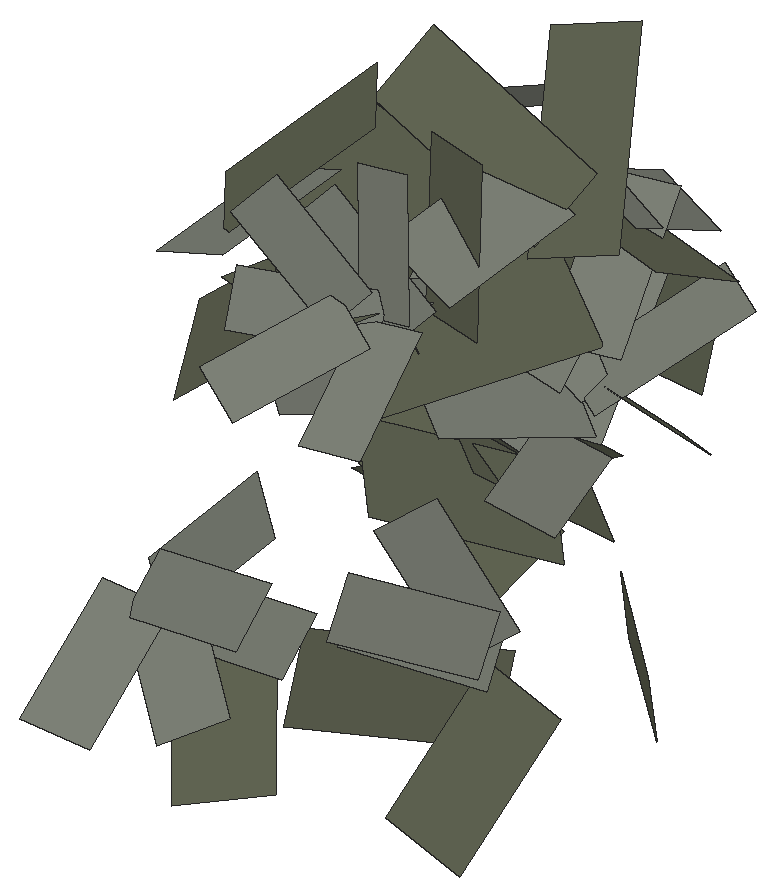
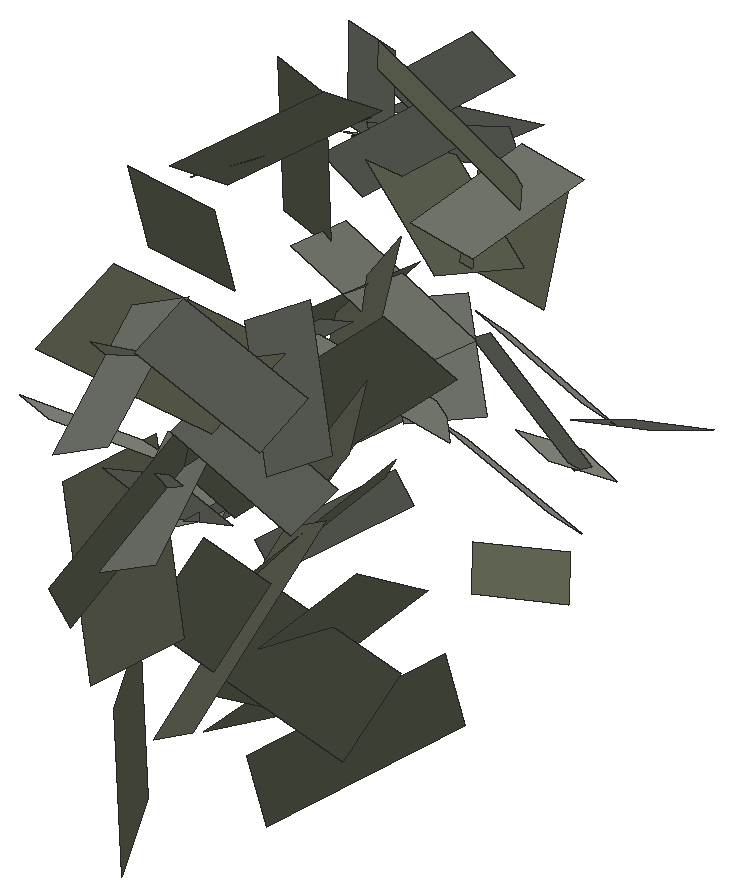
# SketchUp Ruby script. Lengths in inches.
U = 1.inch
M = Sketchup.active_model
def pt(a) = Geom::Point3d.new(a.map { |v| v * U })
def face(e, loops, mat)
  f = e.add_face(loops[0].map { |a| pt(a) })
  loops[1..].each { |l| e.add_face(l.map { |a| pt(a) }).erase! }
  f.material = f.back_material = mat if mat
  f
end
# faces: each face lists its corners as indices into pts; further lists are holes
def faces(e, pts, list, mat = nil) = list.each { |f| face(e, (f[0].is_a?(Array) ? f : [f]).map { |l| l.map { |i| pts[i] } }, mat) }
# xy, xz, yz: faces in a plane at the given z, y or x. An outline is a flat list of corners, or four numbers for a rectangle; further outlines are holes
def ring(l) = l.size == 4 ? [[l[0], l[1]], [l[2], l[1]], [l[2], l[3]], [l[0], l[3]]] : l.each_slice(2).to_a
def flat(e, list, mat, &to3) = list.each { |f| face(e, (f[0].is_a?(Array) ? f : [f]).map { |l| ring(l).map { |u, v| to3.(u, v) } }, mat) }
def xy(e, z, list, mat = nil) = flat(e, list, mat) { |x, y| [x, y, z] }
def xz(e, y, list, mat = nil) = flat(e, list, mat) { |x, z| [x, y, z] }
def yz(e, x, list, mat = nil) = flat(e, list, mat) { |y, z| [x, y, z] }
def lines(e, pts, list) = list.each { |a, b| e.add_line(pt(pts[a]), pt(pts[b])) }
# prism: a flat outline (further loops are holes) pulled along v
def prism(e, loops, v, mat = nil)
  f = face(e, loops, mat); d = Geom::Vector3d.new(v.map { |x| x * U })
  f.pushpull(f.normal.samedirection?(d) ? d.length : -d.length)
end
def box(e, o, s, mat = nil) = prism(e, [[o, [o[0] + s[0], o[1], o[2]], [o[0] + s[0], o[1] + s[1], o[2]], [o[0], o[1] + s[1], o[2]]]], [0, 0, s[2]], mat)
def at(x, y, z, deg = 0) = Geom::Transformation.translation(pt([x, y, z])) * Geom::Transformation.rotation(ORIGIN, Z_AXIS, deg.degrees)
def axes(o, x, y, z) = Geom::Transformation.new([*x, 0, *y, 0, *z, 0, *pt(o).to_a, 1])
def part(name) = M.definitions.add(name)
# library, detail: a bought-in or finely detailed component or shape, given as its bounding box
def library(name, o, s) = part(name).tap { |d| box(d.entities, o, s) }
def detail(e, o, s) = box(e.add_group.entities, o, s)
def put(e, d, t, mat = nil) = e.add_instance(d, t).tap { |i| i.material = mat if mat }
def group(e, t, mat = nil) = e.add_group.tap { |g| g.transformation = t; g.material = mat if mat }.entities
root = M.entities
M.materials.add("viburnumblaasdfas0df1w06d").color = [98, 102, 84]
M.materials.add("viburnumbladsadfasdfad0w122").color = [125, 129, 119]
c1 = part("Component\#315")
p = [[0.25,0,0],[2.05,0.01,0.35],[1.81,4.2,1.66],[0,4.19,1.3125]]
faces(c1.entities,p,[[0,1,2,3]],"viburnumbladsadfasdfad0w122")
c2 = part("viburnumblad2")
put(c2.entities,c1,axes([-19.23,-4.49,-32.18],[83.35428,0,0],[0,79.38502,0],[0,0,83.35428]))
c3 = part("Component\#314")
p = [[0.14,0,0],[2.58,0.05,0.25],[2.44,5.11,2.64],[0,5.05,2.39]]
faces(c3.entities,p,[[0,1,2,3]],"viburnumblaasdfas0df1w06d")
c4 = part("viburnumblad1\#2")
put(c4.entities,c3,axes([-37.25,6.23,19.31],[75.98784,0,0],[0,65.50676,0],[0,0,75.98784]))
put(root,c2,axes([2210.73,337.95,28.6],[-0.01194,-0.00018,-0.00545],[0.00215,-0.01397,-0.00426],[-0.00531,-0.00441,0.0118]))
put(root,c2,axes([2209.76,345.8,24.65],[-0.01038,-0.0062,0.0034],[0.00714,-0.00931,0.00482],[0.00014,0.00586,0.01111]))
put(root,c2,axes([2211.29,330.73,19.29],[-0.01241,-0.00141,0.00136],[-0.00002,-0.00862,-0.00914],[0.00196,-0.00903,0.00851]))
put(root,c4,axes([2212.54,342.4375,14.61],[0.0025,0.01316,0.00583],[-0.01545,-0.00015,0.00696],[0.00546,-0.00635,0.01198]))
put(root,c2,axes([2208.9,345.8,23.2],[-0.00213,-0.01089,0.00325],[0.01232,-0.002,0.0014],[-0.00076,0.00372,0.01198]))
put(root,c4,axes([2212.97,343.62,20.89],[0.00442,0.01183,0.01203],[-0.01827,-0.00182,0.0085],[0.00605,-0.01272,0.01028]))
put(root,c2,axes([2209.18,346.8125,26.02],[-0.00239,-0.01136,0.0048],[0.01232,-0.002,0.0014],[-0.0005,0.00498,0.01153]))
put(root,c4,axes([2209.61,344.26,22.04],[-0.01205,-0.00086,0.01408],[0.00278,-0.02131,0.00108],[0.0139,0.00242,0.01204]))
put(root,c2,axes([2208.75,339.11,23.29],[0.00976,-0.00988,-0.00351],[0.01058,0.00912,0.00376],[-0.00035,-0.00511,0.01338]))
put(root,c4,axes([2208.33,343.53,15.44],[-0.00166,-0.01224,0.00834],[0.01717,-0.00122,0.00163],[-0.00056,0.00844,0.01227]))
put(root,c4,axes([2210.23,336.67,26.12],[-0.00918,-0.00626,-0.00848],[0.01129,-0.01094,-0.00412],[-0.00395,-0.00772,0.00939]))
put(root,c2,axes([2209.25,332.36,19.34],[0.00859,-0.00427,-0.00811],[0.00913,0.005,0.00703],[0.00084,-0.0107,0.00653]))
put(root,c4,axes([2210.1875,335.97,16],[-0.01126,-0.00753,-0.00255],[0.00827,-0.00884,-0.01044],[0.00351,-0.00867,0.01012]))
put(root,c4,axes([2209.0625,335.88,28.07],[0.0077,-0.00971,-0.00377],[0.01191,0.00736,0.00523],[-0.00177,-0.00557,0.01033]))
put(root,c2,axes([2210.55,338.8125,23.09],[-0.01044,-0.00958,-0.00206],[0.0098,-0.01029,-0.00181],[-0.00027,-0.00273,0.01406]))
put(root,c4,axes([2212.72,342.14,11.2],[-0.00036,0.00539,0.01277],[-0.01275,-0.00915,0.0035],[0.00843,-0.01005,0.00448]))
put(root,c2,axes([2210.64,332.47,19.07],[-0.00896,-0.00627,-0.00619],[0.0092,-0.00573,-0.00751],[0.00088,-0.00942,0.00827]))
put(root,c2,axes([2209.64,333.71,18.42],[-0.00025,-0.00716,-0.0097],[0.01356,0.0002,-0.00049],[0.00042,-0.01011,0.00745]))
put(root,c4,axes([2212.88,346.08,15.1],[-0.01278,0.00636,0.00656],[-0.00548,-0.01653,0.00535],[0.00782,0.00178,0.01351]))
put(root,c2,axes([2210.02,338.73,24.99],[-0.00048,-0.01376,-0.00394],[0.01429,-0.00069,0.00066],[-0.00082,-0.00391,0.01375]))
put(root,c2,axes([2210.41,331.39,20.4375],[-0.00026,-0.00745,-0.01011],[0.01255,0.00018,-0.00046],[0.00042,-0.01011,0.00745]))
put(root,c4,axes([2210.32,337.28,26.14],[-0.00628,-0.01206,-0.00336],[0.01448,-0.00668,-0.00311],[0.00091,-0.00388,0.01211]))
put(root,c4,axes([2214.38,342.57,16.61],[-0.00888,0.00849,0.00791],[-0.01054,-0.01309,0.0022],[0.00721,-0.00377,0.01214]))
put(root,c2,axes([2214.66,341.58,19.88],[-0.00337,0.01279,0.00428],[-0.0107,-0.00403,0.00361],[0.00507,-0.00269,0.01202]))
put(root,c2,axes([2214.25,347.25,21.01],[-0.01437,0.00051,0.00412],[0.00025,-0.01266,0.00242],[0.00396,0.00266,0.0135]))
put(root,c2,axes([2214.6,341.2,21.46],[0.0065,0.01157,0.00112],[-0.00968,0.00489,0.00566],[0.0049,-0.00389,0.01176]))
put(root,c4,axes([2214.3125,348.18,19.03],[-0.00461,0.01011,0.01059],[-0.01024,-0.0125,0.00748],[0.01168,-0.00415,0.00905]))
put(root,c2,axes([2215.53,333.41,26.72],[-0.00143,0.00635,0.00868],[-0.0108,-0.00196,-0.00037],[0.00136,-0.00839,0.00553]))
put(root,c2,axes([2214.72,332.47,27.625],[0.00668,0.00514,0.00687],[-0.00864,0.00277,0.00603],[0.00109,-0.00897,0.00475]))
put(root,c2,axes([2215.77,340.6875,22.85],[-0.00323,0.01225,0.0041],[-0.01189,-0.00447,0.00401],[0.00507,-0.00269,0.01202]))
put(root,c2,axes([2215.05,334.64,26.29],[0.00642,0.00493,0.0066],[-0.00933,0.00299,0.00651],[0.00109,-0.00897,0.00475]))
put(root,c4,axes([2215.46,342.66,23.27],[-0.01126,0.00378,0.01091],[-0.00977,-0.0152,-0.00482],[0.00789,-0.0086,0.01113]))
put(root,c2,axes([2213.59,342.32,20.49],[0.01096,0.00423,-0.00348],[-0.00277,0.01177,0.00559],[0.00527,-0.00421,0.01149]))
put(root,c2,axes([2216.04,341.79,21.22],[-0.01106,0.00576,0.00468],[-0.00631,-0.01247,0.00042],[0.00435,-0.00178,0.01246]))
put(root,c4,axes([2210.71,345.8125,25.33],[-0.00321,-0.01557,0.00645],[0.01613,-0.00714,-0.00921],[0.00952,0.00374,0.01377]))
put(root,c2,axes([2216.11,332.45,27.57],[-0.00871,0.00384,0.00541],[-0.00663,-0.00614,-0.00616],[0.00084,-0.00787,0.00624]))
put(root,c4,axes([2216.52,339.28,27.64],[0.00193,0.01121,0.0059],[-0.01433,0.00039,0.00396],[0.00283,-0.0062,0.01085]))
put(root,c2,axes([2215.42,347.6875,24.33],[-0.01376,0.00048,0.00394],[0.00028,-0.01406,0.00269],[0.00396,0.00266,0.0135]))
put(root,c2,axes([2216.15,337.25,15.79],[-0.00143,0.00682,0.00818],[-0.0095,-0.00594,0.0033],[0.00662,-0.0068,0.00682]))
put(root,c4,axes([2214.86,341.45,12.95],[-0.00935,-0.00415,0.00773],[-0.00246,-0.01147,-0.00913],[0.00851,-0.00702,0.00652]))
put(root,c4,axes([2213.29,347.73,17.48],[-0.01204,-0.00702,0.00725],[0.00958,-0.01547,0.00093],[0.0058,0.00442,0.01392]))
put(root,c4,axes([2215.11,340.85,25.74],[0.01317,0.00353,0.00249],[-0.00497,0.01356,0.00706],[-0.00054,-0.00655,0.0122]))
put(root,c2,axes([2214.54,341.65,23.46],[0.01242,0.00411,-0.00252],[-0.00277,0.01177,0.00559],[0.00395,-0.00468,0.01183]))
put(root,c2,axes([2214.62,333.91,27.39],[0.01089,0.00092,0.00104],[-0.00149,0.00552,0.00975],[0.0002,-0.00927,0.00435]))
put(root,c4,axes([2214.62,337.34,25.71],[0.0117,-0.0027,-0.00014],[0.00141,0.00653,0.01192],[-0.00257,-0.00994,0.00471]))
put(root,c4,axes([2213.39,346.59,11.49],[-0.00616,-0.00011,0.01357],[0.00475,-0.0165,0.00202],[0.01294,0.00445,0.00591]))
put(root,c2,axes([2215.59,343,19.93],[-0.01192,-0.00395,0.00242],[0.00393,-0.01356,-0.00276],[0.00316,-0.0017,0.01283]))
put(root,c2,axes([2216.06,336.2,16.96],[0.00667,0.00821,0.00496],[-0.00717,0.00016,0.00937],[0.00645,-0.00831,0.00509]))
put(root,c2,axes([2216.97,339.66,28.64],[-0.01426,0.00099,0.00559],[-0.00302,-0.01157,-0.00566],[0.00428,-0.00706,0.01216]))
put(root,c2,axes([2216.55,333.99,27.49],[-0.01089,-0.00092,-0.00104],[0.00144,-0.00742,-0.00803],[-0.00015,-0.00772,0.00646]))
put(root,c2,axes([2217.42,335.31,17.37],[-0.00083,0.00664,0.00958],[-0.0095,-0.00594,0.0033],[0.00675,-0.00756,0.00582]))
put(root,c2,axes([2214.16,342.92,22.08],[0.01106,-0.00576,-0.00468],[0.00696,0.01121,0.00265],[0.00276,-0.0046,0.01219]))
